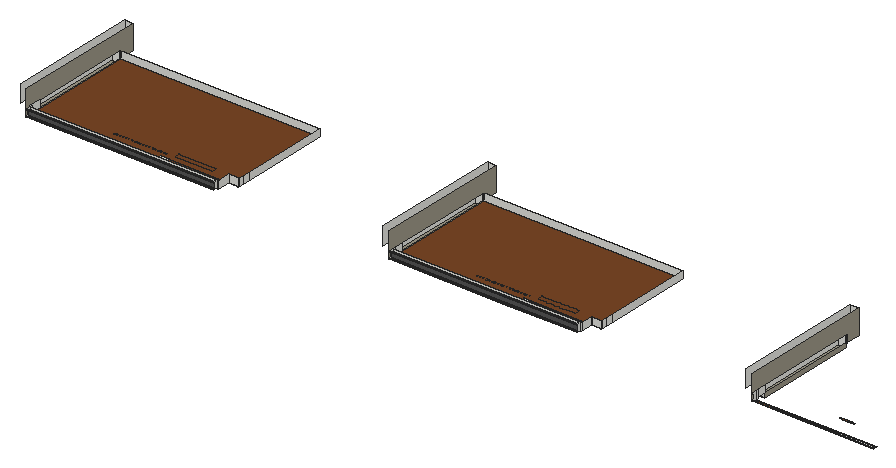
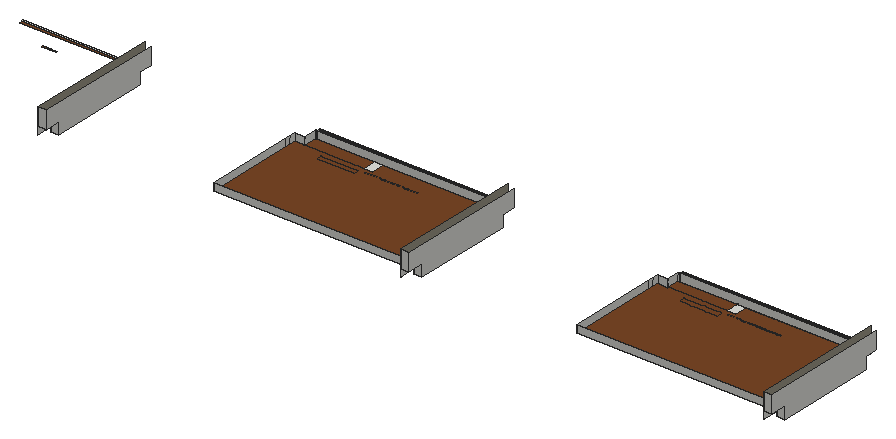
# SketchUp Ruby script. Lengths in inches.
U = 1.inch
M = Sketchup.active_model
def pt(a) = Geom::Point3d.new(a.map { |v| v * U })
def face(e, loops, mat)
  f = e.add_face(loops[0].map { |a| pt(a) })
  loops[1..].each { |l| e.add_face(l.map { |a| pt(a) }).erase! }
  f.material = f.back_material = mat if mat
  f
end
# faces: each face lists its corners as indices into pts; further lists are holes
def faces(e, pts, list, mat = nil) = list.each { |f| face(e, (f[0].is_a?(Array) ? f : [f]).map { |l| l.map { |i| pts[i] } }, mat) }
# xy, xz, yz: faces in a plane at the given z, y or x. An outline is a flat list of corners, or four numbers for a rectangle; further outlines are holes
def ring(l) = l.size == 4 ? [[l[0], l[1]], [l[2], l[1]], [l[2], l[3]], [l[0], l[3]]] : l.each_slice(2).to_a
def flat(e, list, mat, &to3) = list.each { |f| face(e, (f[0].is_a?(Array) ? f : [f]).map { |l| ring(l).map { |u, v| to3.(u, v) } }, mat) }
def xy(e, z, list, mat = nil) = flat(e, list, mat) { |x, y| [x, y, z] }
def xz(e, y, list, mat = nil) = flat(e, list, mat) { |x, z| [x, y, z] }
def yz(e, x, list, mat = nil) = flat(e, list, mat) { |y, z| [x, y, z] }
def lines(e, pts, list) = list.each { |a, b| e.add_line(pt(pts[a]), pt(pts[b])) }
# prism: a flat outline (further loops are holes) pulled along v
def prism(e, loops, v, mat = nil)
  f = face(e, loops, mat); d = Geom::Vector3d.new(v.map { |x| x * U })
  f.pushpull(f.normal.samedirection?(d) ? d.length : -d.length)
end
def box(e, o, s, mat = nil) = prism(e, [[o, [o[0] + s[0], o[1], o[2]], [o[0] + s[0], o[1] + s[1], o[2]], [o[0], o[1] + s[1], o[2]]]], [0, 0, s[2]], mat)
def at(x, y, z, deg = 0) = Geom::Transformation.translation(pt([x, y, z])) * Geom::Transformation.rotation(ORIGIN, Z_AXIS, deg.degrees)
def axes(o, x, y, z) = Geom::Transformation.new([*x, 0, *y, 0, *z, 0, *pt(o).to_a, 1])
def part(name) = M.definitions.add(name)
# library, detail: a bought-in or finely detailed component or shape, given as its bounding box
def library(name, o, s) = part(name).tap { |d| box(d.entities, o, s) }
def detail(e, o, s) = box(e.add_group.entities, o, s)
def put(e, d, t, mat = nil) = e.add_instance(d, t).tap { |i| i.material = mat if mat }
def group(e, t, mat = nil) = e.add_group.tap { |g| g.transformation = t; g.material = mat if mat }.entities
root = M.entities
M.materials.add("[Color M05]").color = [86, 86, 86]
M.materials.add("[Concrete Tile]").color = [155, 150, 134]
M.materials.add("[Wood Veneer 01]").color = [120, 70, 37]
xy(root,254.125,[[352.17,877.14,352.17,1122.97,372.3,1122.97,372.92,877.14],[1232.12,877.14,1232.12,1122.97,1252.24,1122.97,1252.87,877.14],[2112.0625,877.14,2112.0625,1122.97,2132.1875,1122.97,2132.8125,877.14]],"[Concrete Tile]")
xy(root,264.75,[[667.84,840.97,687.49,845.35],[1547.79,840.97,1567.4375,845.35],[667.84,845.35,687.49,877.14],[827.91,845.35,832,846.1],[1547.79,845.35,1567.4375,877.14],
  [1707.86,845.35,1711.94,846.1],[832,877.14,857.125,877.51],[1711.94,877.14,1737.07,877.51]])
xy(root,264.75,[[374.86,837.03,667.84,845.35],[667.84,837.03,687.49,840.97],[687.49,837.03,827.91,845.35],[1254.81,837.03,1547.79,845.35],[1547.79,837.03,1567.4375,840.97],
  [1567.4375,837.03,1707.86,845.35],[2134.75,837.03,2427.73,845.35],[[374.86,845.35,374.86,850.97,372.92,850.97,372.92,877.14,372.3,1122.97,372.3,1160.85,372.92,1160.85,372.92,1122.97,857.125,1122.97,857.125,877.51,832,877.51,832,877.14,667.84,877.14,667.84,845.35],[687.6875,890.39,782.75,905.7],[650.22,888.83,655.63,890.39],[664.22,888.83,669.63,890.39],[657.22,888.83,662.63,890.39],[671.22,888.83,676.63,890.39],[643.22,888.83,648.63,890.39],[636.22,888.83,641.63,890.39],[545.16,888.95,550.57,890.39],[580.22,888.95,585.63,890.39],[601.22,888.95,606.63,890.39],[552.22,888.95,557.63,890.39],[629.22,888.95,634.63,890.39],[622.22,888.95,627.63,890.39],[608.22,888.95,613.63,890.39],[615.22,888.95,620.63,890.39],[559.22,888.95,564.63,890.39],[573.22,888.95,578.63,890.39],[587.22,888.95,592.63,890.39],[594.22,888.95,599.63,890.39],[566.22,888.95,571.63,890.39]],[687.49,845.35,687.49,877.14,832,877.14,832,846.1,827.91,846.1,827.91,845.35],[[1254.81,845.35,1254.81,850.97,1252.87,850.97,1252.87,877.14,1252.24,1122.97,1252.24,1160.85,1252.87,1160.85,1252.87,1122.97,1737.07,1122.97,1737.07,877.51,1711.94,877.51,1711.94,877.14,1547.79,877.14,1547.79,845.35],[1567.63,890.39,1662.7,905.7],[1530.16,888.83,1535.58,890.39],[1544.16,888.83,1549.58,890.39],[1537.16,888.83,1542.58,890.39],[1551.16,888.83,1556.58,890.39],[1523.16,888.83,1528.58,890.39],[1516.16,888.83,1521.58,890.39],[1425.1,888.95,1430.52,890.39],[1460.16,888.95,1465.58,890.39],[1481.16,888.95,1486.58,890.39],[1432.16,888.95,1437.58,890.39],[1509.16,888.95,1514.58,890.39],[1502.16,888.95,1507.58,890.39],[1488.16,888.95,1493.58,890.39],[1495.16,888.95,1500.58,890.39],[1439.16,888.95,1444.58,890.39],[1453.16,888.95,1458.58,890.39],[1467.16,888.95,1472.58,890.39],[1474.16,888.95,1479.58,890.39],[1446.16,888.95,1451.58,890.39]],
  [1567.4375,845.35,1567.4375,877.14,1711.94,877.14,1711.94,846.1,1707.86,846.1,1707.86,845.35],[636.22,888.83,641.63,890.39],[643.22,888.83,648.63,890.39],[650.22,888.83,655.63,890.39],[657.22,888.83,662.63,890.39],
  [664.22,888.83,669.63,890.39],[671.22,888.83,676.63,890.39],[1516.16,888.83,1521.58,890.39],[1523.16,888.83,1528.58,890.39],[1530.16,888.83,1535.58,890.39],
  [1537.16,888.83,1542.58,890.39],[1544.16,888.83,1549.58,890.39],[1551.16,888.83,1556.58,890.39],[545.16,888.95,550.57,890.39],[552.22,888.95,557.63,890.39],
  [559.22,888.95,564.63,890.39],[566.22,888.95,571.63,890.39],[573.22,888.95,578.63,890.39],[580.22,888.95,585.63,890.39],[587.22,888.95,592.63,890.39],
  [594.22,888.95,599.63,890.39],[601.22,888.95,606.63,890.39],[608.22,888.95,613.63,890.39],[615.22,888.95,620.63,890.39],[622.22,888.95,627.63,890.39],
  [629.22,888.95,634.63,890.39],[1425.1,888.95,1430.52,890.39],[1432.16,888.95,1437.58,890.39],[1439.16,888.95,1444.58,890.39],[1446.16,888.95,1451.58,890.39],
  [1453.16,888.95,1458.58,890.39],[1460.16,888.95,1465.58,890.39],[1467.16,888.95,1472.58,890.39],[1474.16,888.95,1479.58,890.39],[1481.16,888.95,1486.58,890.39],
  [1488.16,888.95,1493.58,890.39],[1495.16,888.95,1500.58,890.39],[1502.16,888.95,1507.58,890.39],[1509.16,888.95,1514.58,890.39],[2305.05,888.95,2310.46,890.39],
  [2312.11,888.95,2317.52,890.39],[2319.11,888.95,2324.52,890.39],[2326.11,888.95,2331.52,890.39],[2333.11,888.95,2338.52,890.39],[687.6875,890.39,782.75,905.7],
  [1567.63,890.39,1662.7,905.7]],"[Wood Veneer 01]")
xy(root,266.9375,[[374.86,837.03,667.84,840.97],[667.84,837.03,687.49,840.97],[687.49,837.03,827.91,840.97],[1254.81,837.03,1547.79,840.97],[1547.79,837.03,1567.4375,840.97],
  [1567.4375,837.03,1707.86,840.97],[2134.75,837.03,2427.73,840.97]])
xy(root,280.5625,[[374.86,837.03,827.91,840.97],[1254.81,837.03,1707.86,840.97]])
xz(root,837.03,[[374.86,264.75,827.91,266.9375],[1254.81,264.75,1707.86,266.9375],[374.86,280.5625,827.91,282.75],[1254.81,280.5625,1707.86,282.75]],"[Color M05]")
xz(root,840.97,[[374.86,266.9375,827.91,280.5625],[1254.81,266.9375,1707.86,280.5625]],"[Color M05]")
xz(root,845.35,[[374.86,264.75,827.91,282.75],[827.91,264.75,832,282.75],[1254.81,264.75,1707.86,282.75],[1707.86,264.75,1711.94,282.75]])
xz(root,850.97,[[372.92,264.75,374.86,282.75],[1252.87,264.75,1254.81,282.75],[2132.8125,264.75,2134.75,282.75]])
xz(root,877.14,[[352.17,254.125,372.92,282.75],[1232.12,254.125,1252.87,282.75],[2112.0625,254.125,2132.8125,282.75],[832,264.75,857.125,282.75],[1711.94,264.75,1737.07,282.75]])
xz(root,877.51,[[832,264.75,857.125,282.75],[1711.94,264.75,1737.07,282.75]])
xz(root,1122.97,[[352.17,254.125,372.3,282.75],[1232.12,254.125,1252.24,282.75],[2112.0625,254.125,2132.1875,282.75],[372.92,264.75,374.86,282.75],[374.86,264.75,857.125,282.75],
  [1252.87,264.75,1254.81,282.75],[1254.81,264.75,1737.07,282.75],[2132.8125,264.75,2134.75,282.75]])
xz(root,1160.85,[[372.3,264.75,372.3,282.75,352.17,282.75,352.17,324.5625,372.92,324.5625,372.92,264.75],[1252.24,264.75,1252.24,282.75,1232.12,282.75,1232.12,324.5625,1252.87,324.5625,1252.87,264.75],[2132.1875,264.75,2132.1875,282.75,2112.0625,282.75,2112.0625,324.5625,2132.8125,324.5625,2132.8125,264.75]])
yz(root,352.17,[[877.14,254.125,877.14,282.75,845.35,282.75,845.35,324.5625,1160.85,324.5625,1160.85,282.75,1122.97,282.75,1122.97,254.125]])
yz(root,372.3,[[1122.97,264.75,1160.85,282.75]])
yz(root,372.92,[[845.35,264.75,850.97,282.75],[850.97,264.75,877.14,282.75]])
yz(root,372.92,[[837.03,264.75,845.35,264.75,845.35,282.75,1122.97,282.75,1122.97,264.75,1160.85,264.75,1160.85,324.5625,837.03,324.5625]],"[Concrete Tile]")
yz(root,374.86,[[837.03,264.75,837.03,266.9375,840.97,266.9375,840.97,280.5625,837.03,280.5625,837.03,282.75,845.35,282.75,845.35,264.75],[845.35,264.75,850.97,282.75]])
yz(root,827.91,[[837.03,264.75,840.97,266.9375],[840.97,264.75,845.35,282.75],[837.03,280.5625,840.97,282.75]])
yz(root,832,[[845.35,264.75,846.1,282.75],[846.1,264.75,877.14,282.75],[877.14,264.75,877.51,282.75]])
yz(root,857.125,[[877.14,264.75,877.51,282.75],[877.51,264.75,890.39,282.75],[890.39,264.75,905.7,282.75],[905.7,264.75,1122.97,282.75]])
yz(root,1232.12,[[877.14,254.125,877.14,282.75,845.35,282.75,845.35,324.5625,1160.85,324.5625,1160.85,282.75,1122.97,282.75,1122.97,254.125]])
yz(root,1252.24,[[1122.97,264.75,1160.85,282.75]])
yz(root,1252.87,[[845.35,264.75,850.97,282.75],[850.97,264.75,877.14,282.75]])
yz(root,1252.87,[[837.03,264.75,845.35,264.75,845.35,282.75,1122.97,282.75,1122.97,264.75,1160.85,264.75,1160.85,324.5625,837.03,324.5625]],"[Concrete Tile]")
yz(root,1254.81,[[837.03,264.75,837.03,266.9375,840.97,266.9375,840.97,280.5625,837.03,280.5625,837.03,282.75,845.35,282.75,845.35,264.75],[845.35,264.75,850.97,282.75]])
yz(root,1707.86,[[837.03,264.75,840.97,266.9375],[840.97,264.75,845.35,282.75],[837.03,280.5625,840.97,282.75]])
yz(root,1711.94,[[845.35,264.75,846.1,282.75],[846.1,264.75,877.14,282.75],[877.14,264.75,877.51,282.75]])
yz(root,1737.07,[[877.14,264.75,877.51,282.75],[877.51,264.75,890.39,282.75],[890.39,264.75,905.7,282.75],[905.7,264.75,1122.97,282.75]])
yz(root,2112.0625,[[877.14,254.125,877.14,282.75,845.35,282.75,845.35,324.5625,1160.85,324.5625,1160.85,282.75,1122.97,282.75,1122.97,254.125]])
yz(root,2132.1875,[[1122.97,264.75,1160.85,282.75]])
yz(root,2132.8125,[[845.35,264.75,850.97,282.75],[850.97,264.75,877.14,282.75]])
yz(root,2132.8125,[[837.03,264.75,845.35,264.75,845.35,282.75,1122.97,282.75,1122.97,264.75,1160.85,264.75,1160.85,324.5625,837.03,324.5625]],"[Concrete Tile]")
yz(root,2134.75,[[837.03,264.75,837.03,266.9375,840.97,266.9375,840.97,280.5625,837.03,280.5625,837.03,282.75,845.35,282.75,845.35,264.75],[845.35,264.75,850.97,282.75]])
p = [[372.3,1122.97,264.75],[372.92,877.14,264.75],[372.92,877.14,254.125],[372.3,1122.97,254.125],[1252.24,1122.97,264.75],[1252.87,877.14,264.75],
  [1252.87,877.14,254.125],[1252.24,1122.97,254.125],[2132.1875,1122.97,264.75],[2132.8125,877.14,264.75],[2132.8125,877.14,254.125],[2132.1875,1122.97,254.125]]
faces(root,p,[[0,1,2,3],[4,5,6,7],[8,9,10,11]],"[Concrete Tile]")
